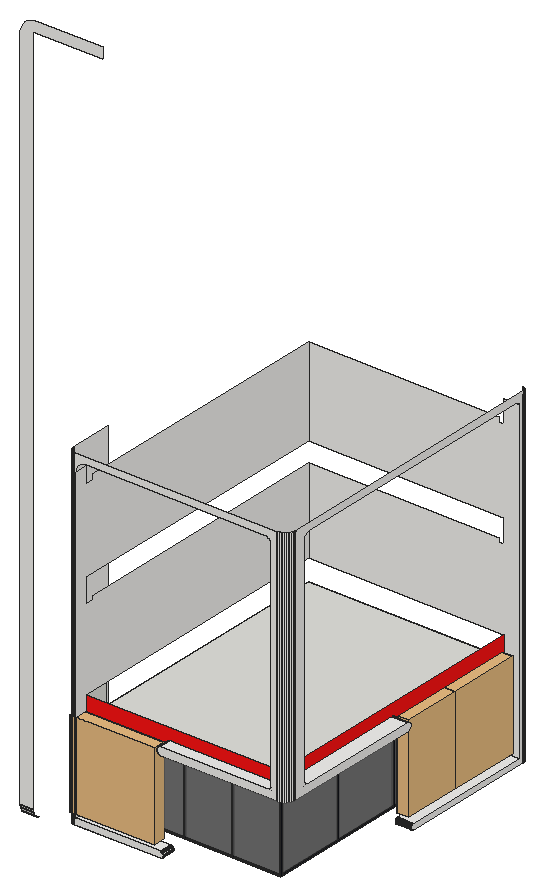
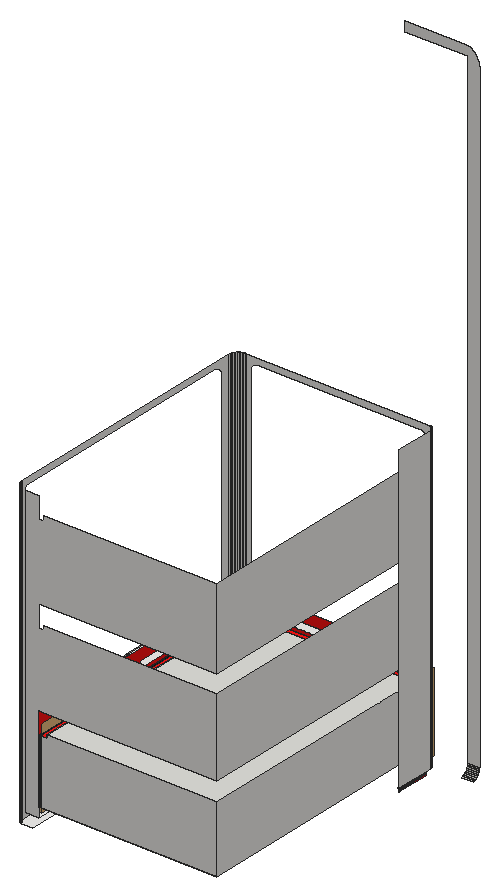
# SketchUp Ruby script. Lengths in inches.
U = 1.inch
M = Sketchup.active_model
def pt(a) = Geom::Point3d.new(a.map { |v| v * U })
def face(e, loops, mat)
  f = e.add_face(loops[0].map { |a| pt(a) })
  loops[1..].each { |l| e.add_face(l.map { |a| pt(a) }).erase! }
  f.material = f.back_material = mat if mat
  f
end
# faces: each face lists its corners as indices into pts; further lists are holes
def faces(e, pts, list, mat = nil) = list.each { |f| face(e, (f[0].is_a?(Array) ? f : [f]).map { |l| l.map { |i| pts[i] } }, mat) }
# xy, xz, yz: faces in a plane at the given z, y or x. An outline is a flat list of corners, or four numbers for a rectangle; further outlines are holes
def ring(l) = l.size == 4 ? [[l[0], l[1]], [l[2], l[1]], [l[2], l[3]], [l[0], l[3]]] : l.each_slice(2).to_a
def flat(e, list, mat, &to3) = list.each { |f| face(e, (f[0].is_a?(Array) ? f : [f]).map { |l| ring(l).map { |u, v| to3.(u, v) } }, mat) }
def xy(e, z, list, mat = nil) = flat(e, list, mat) { |x, y| [x, y, z] }
def xz(e, y, list, mat = nil) = flat(e, list, mat) { |x, z| [x, y, z] }
def yz(e, x, list, mat = nil) = flat(e, list, mat) { |y, z| [x, y, z] }
def lines(e, pts, list) = list.each { |a, b| e.add_line(pt(pts[a]), pt(pts[b])) }
# prism: a flat outline (further loops are holes) pulled along v
def prism(e, loops, v, mat = nil)
  f = face(e, loops, mat); d = Geom::Vector3d.new(v.map { |x| x * U })
  f.pushpull(f.normal.samedirection?(d) ? d.length : -d.length)
end
def box(e, o, s, mat = nil) = prism(e, [[o, [o[0] + s[0], o[1], o[2]], [o[0] + s[0], o[1] + s[1], o[2]], [o[0], o[1] + s[1], o[2]]]], [0, 0, s[2]], mat)
def at(x, y, z, deg = 0) = Geom::Transformation.translation(pt([x, y, z])) * Geom::Transformation.rotation(ORIGIN, Z_AXIS, deg.degrees)
def axes(o, x, y, z) = Geom::Transformation.new([*x, 0, *y, 0, *z, 0, *pt(o).to_a, 1])
def part(name) = M.definitions.add(name)
# library, detail: a bought-in or finely detailed component or shape, given as its bounding box
def library(name, o, s) = part(name).tap { |d| box(d.entities, o, s) }
def detail(e, o, s) = box(e.add_group.entities, o, s)
def put(e, d, t, mat = nil) = e.add_instance(d, t).tap { |i| i.material = mat if mat }
def group(e, t, mat = nil) = e.add_group.tap { |g| g.transformation = t; g.material = mat if mat }.entities
root = M.entities
M.materials.add("Generic").color = [242, 241, 238]
M.materials.add("Heather_Band").color = [255, 20, 20]
M.materials.add("Lisanne_Bandana").color = [222, 18, 34]
M.materials.add("{045efeae-c101-a24d-bd9b-6f5600100adb}").color = [102, 102, 102]
M.materials["{045efeae-c101-a24d-bd9b-6f5600100adb}"].alpha = 0.7
M.materials.add("{16756a1b-d383-d94f-ad82-104813d2624f}").color = [19, 21, 27]
c1 = library("Shrub+_Grass",[-121.83,-22.34,0],[123.96,19.94,123.95])
c2 = part("Furniture_0DcpanrIvuI8n_9Ae92L5A")
g1 = group(c2.entities,at(0,0,0))
box(g1,[-19.29,-0.2,0.39],[38.58,0.4,83.86],"{045efeae-c101-a24d-bd9b-6f5600100adb}")
g2 = group(c2.entities,at(0,0,0))
box(g2,[-19.68,-0.59,63.39],[39.36,1.18,0.39],"{16756a1b-d383-d94f-ad82-104813d2624f}")
box(g2,[-19.68,-0.59,42.52],[39.36,1.18,0.39],"{16756a1b-d383-d94f-ad82-104813d2624f}")
box(g2,[-19.68,-0.59,21.26],[39.36,1.18,0.39],"{16756a1b-d383-d94f-ad82-104813d2624f}")
xy(g2,0,[[-19.68,-0.59,19.68,0.59]],"{16756a1b-d383-d94f-ad82-104813d2624f}")
xy(g2,0.39,[[-19.68,-0.59,-19.29,0.59],[-19.68,-0.59,19.68,0.59],[19.29,-0.59,19.68,0.59]],"{16756a1b-d383-d94f-ad82-104813d2624f}")
xy(g2,84.25,[[-19.68,-0.59,19.68,0.59]],"{16756a1b-d383-d94f-ad82-104813d2624f}")
xy(g2,84.65,[[-19.68,-0.59,-19.29,0.59],[-19.68,-0.59,19.68,0.59],[19.29,-0.59,19.68,0.59]],"{16756a1b-d383-d94f-ad82-104813d2624f}")
xz(g2,-0.59,[[-19.68,0,19.68,0.39],[-19.68,0.39,-19.29,84.65],[19.29,0.39,19.68,84.65],[-19.68,84.25,19.68,84.65]],"{16756a1b-d383-d94f-ad82-104813d2624f}")
xz(g2,0.59,[[-19.68,0,19.68,0.39],[-19.68,0.39,-19.29,84.65],[19.29,0.39,19.68,84.65],[-19.68,84.25,19.68,84.65]],"{16756a1b-d383-d94f-ad82-104813d2624f}")
yz(g2,-19.68,[[-0.59,0,0.59,0.39],[-0.59,0.39,0.59,84.65],[-0.59,84.25,0.59,84.65]],"{16756a1b-d383-d94f-ad82-104813d2624f}")
yz(g2,-19.29,[[-0.59,0.39,0.59,84.65]],"{16756a1b-d383-d94f-ad82-104813d2624f}")
yz(g2,19.29,[[-0.59,0.39,0.59,84.65]],"{16756a1b-d383-d94f-ad82-104813d2624f}")
yz(g2,19.68,[[-0.59,0,0.59,0.39],[-0.59,0.39,0.59,84.65],[-0.59,84.25,0.59,84.65]],"{16756a1b-d383-d94f-ad82-104813d2624f}")
c3 = part("Glass+Window")
put(c3.entities,c2,at(0,0,-42.32))
xy(root,260.43,[[144.5,115.9,143.11,115.99,141.75,116.26,140.43,116.71,139.18,117.33,138.02,118.1,136.98,119.02,136.06,120.0625,135.28,121.22,134.67,122.47,134.22,123.79,133.95,125.15,133.86,126.54,133.86,200.9,136.89,200.9,136.89,137.375,291.875,137.375,291.875,115.9],[482.71,389.19,482.71,632.34,503.14,632.34,504.14,632.27,505.13,632.08,506.08,631.75,506.98,631.31,507.82,630.75,508.58,630.08,509.24,629.33,509.8,628.49,510.25,627.59,510.57,626.63,510.77,625.65,510.83,624.64,510.83,389.19]],"Generic")
xy(root,270.68,[[482.71,389.19,510.83,617.58]],"Generic")
xy(root,270.88,[[145.77,115.9,291.875,137.375]],"Generic")
xy(root,289.68,[[145.77,137.375,479.5,137.375,479.92,137.4,480.33,137.49,480.73,137.62,481.11,137.81,481.46,138.04,481.77,138.32,482.05,138.63,482.28,138.98,482.47,139.36,482.6,139.75,482.6875,140.17,482.71,140.59,482.71,617.58,145.77,617.58]])
xy(root,412.09,[[145.77,137.375,145.77,151.79,468.61,151.79,468.61,617.58,482.71,617.58,482.71,137.375]],"Heather_Band")
xy(root,416.32,[[145.77,151.79,468.61,617.58]])
xy(root,418.86,[[292.72,115.9,292.72,137.375,482.71,137.375,482.71,374.78,510.83,374.78,510.83,134.62,510.67,132.17,510.2,129.77,509.41,127.45,508.33,125.26,506.97,123.22,505.35,121.38,503.51,119.77,501.48,118.41,499.28,117.33,496.96,116.54,494.5625,116.0625,492.12,115.9]],"Generic")
xy(root,432.33,[[292.72,115.9,477.39,137.375],[482.71,160.35,510.83,374.78]],"Generic")
xz(root,96.24,[[65.42,274,87.56,274,87.56,1474.125,207.5,1474.125,207.5,1492.875,95.21,1492.875,91.33,1492.62,87.5,1491.86,83.8125,1490.61,80.32,1488.88,77.08,1486.72,74.15,1484.15,71.58,1481.22,69.41,1477.98,67.6875,1474.48,66.4375,1470.79,65.68,1466.97,65.42,1463.08]],"Generic")
xz(root,115.9,[[144.5,260.43,291.875,260.43,292.42,260.46,292.96,260.55,293.49,260.6875,294,260.89,294.49,261.13,294.95,261.43,295.37,261.78,295.76,262.16,296.1,262.59,296.4,263.05,296.65,263.53,296.84,264.04,296.99,264.57,297.07,265.11,297.1,265.66,297.07,266.2,296.99,266.74,296.84,267.27,296.65,267.78,296.4,268.27,296.1,268.73,295.76,269.15,295.37,269.54,294.95,269.88,294.49,270.18,294,270.43,293.49,270.625,292.96,270.77,292.42,270.85,291.875,270.88,145.77,270.88,145.77,805.02,145.93,807.42,146.39,809.78,147.17,812.05,148.23,814.21,149.5625,816.21,151.15,818.01,152.95,819.6,154.95,820.93,157.11,821.99,159.38,822.77,161.74,823.23,164.14,823.39,470.91,823.39,472.35,823.3,473.77,823.04,475.14,822.61,476.46,822.02,477.69,821.27,478.82,820.37,479.84,819.35,480.72,818.21,481.46,816.97,482.04,815.65,482.46,814.27,482.71,812.85,482.71,439.07,482.63,438.03,482.4,437,482.01,436.03,481.48,435.12,480.82,434.3,480.04,433.6,479.17,433.01,478.21,432.57,477.39,432.33,292.72,432.33,292.02,432.29,291.32,432.18,290.64,432,289.98,431.75,289.35,431.43,288.76,431.04,288.21,430.6,287.71,430.1,287.27,429.55,286.89,428.96,286.57,428.33,286.3125,427.68,286.13,426.99,286.02,426.3,285.98,425.59,286.02,424.89,286.13,424.19,286.3125,423.51,286.57,422.85,286.89,422.23,287.27,421.63,287.71,421.09,288.21,420.59,288.76,420.14,289.35,419.76,289.98,419.4375,290.64,419.1875,291.32,419,292.02,418.89,292.72,418.86,492.12,418.86,492.12,835.52,144.5,835.52]],"Generic")
xz(root,137.375,[[145.77,412.09,482.71,412.09,482.71,418.86,292.72,418.86,292.02,418.89,291.32,419,290.64,419.1875,289.98,419.4375,289.35,419.76,288.76,420.14,288.21,420.59,287.71,421.09,287.27,421.63,286.89,422.23,286.57,422.85,286.3125,423.51,286.13,424.19,286.02,424.89,285.98,425.59,286.02,426.3,286.13,426.99,286.3125,427.68,286.57,428.33,286.89,428.96,287.27,429.55,287.71,430.1,288.21,430.6,288.76,431.04,289.35,431.43,289.98,431.75,290.64,432,291.32,432.18,292.02,432.29,292.72,432.33,477.39,432.33,478.21,432.57,479.17,433.01,480.04,433.6,480.82,434.3,481.48,435.12,482.01,436.03,482.4,437,482.63,438.03,482.71,439.07,482.71,452.24,145.77,452.24]],"Heather_Band")
xz(root,151.79,[[145.77,412.09,468.61,416.32]])
xz(root,617.58,[[482.71,270.68,510.83,270.68,510.83,817.55,482.71,817.55,482.71,777.77,474.55,777.77,474.55,786.62,145.77,786.62,145.77,633.64,482.71,633.64,482.71,592.96,474.55,592.96,474.55,599,145.77,599,145.77,452.24,482.71,452.24,482.71,412.09,468.61,412.09,468.61,416.32,145.77,416.32,145.77,289.68,482.71,289.68]],"Generic")
yz(root,133.86,[[126.54,260.43,200.9,835.52]],"Generic")
yz(root,133.86,[[137.375,255.93,200.9,255.95],[137.375,255.95,200.9,257.23]],"Lisanne_Bandana")
yz(root,145.77,[[137.375,412.09,151.79,412.09,151.79,416.32,181.19,416.32,180.67,452.24,137.375,452.24]])
yz(root,145.77,[[115.9,270.88,137.375,270.88,137.375,289.68,617.58,289.68,617.58,416.32,151.79,416.32,151.79,412.09,137.375,412.09,137.375,452.24,617.58,452.24,617.58,599,151.79,599,151.79,592.96,137.375,592.96,137.375,633.64,617.58,633.64,617.58,786.62,151.79,786.62,151.79,777.77,137.375,777.77,137.375,805.02,115.9,805.02]],"Generic")
yz(root,468.61,[[151.79,412.09,617.58,416.32]])
yz(root,482.71,[[137.375,412.09,617.58,412.09,617.58,452.24,150.43,452.24,150.43,444.64,150.51,443.22,150.75,441.82,151.15,440.45,151.69,439.14,152.39,437.89,153.22,436.74,154.17,435.68,155.24,434.74,156.41,433.92,157.66,433.24,158.98,432.71,160.35,432.33,374.78,432.33,375.48,432.29,376.18,432.18,376.86,432,377.52,431.75,378.15,431.43,378.74,431.04,379.29,430.6,379.78,430.1,380.23,429.55,380.61,428.96,380.93,428.33,381.18,427.68,381.37,426.99,381.48,426.3,381.51,425.59,381.48,424.89,381.37,424.19,381.18,423.51,380.93,422.85,380.61,422.23,380.23,421.63,379.78,421.09,379.29,420.59,378.74,420.14,378.15,419.76,377.52,419.4375,376.86,419.1875,376.18,419,375.48,418.89,374.78,418.86,137.375,418.86]],"Heather_Band")
yz(root,510.83,[[389.19,260.43,624.64,260.43,624.64,835.52,134.62,835.52,134.62,418.86,374.78,418.86,375.48,418.89,376.18,419,376.86,419.1875,377.52,419.4375,378.15,419.76,378.74,420.14,379.29,420.59,379.78,421.09,380.23,421.63,380.61,422.23,380.93,422.85,381.18,423.51,381.37,424.19,381.48,424.89,381.51,425.59,381.48,426.3,381.37,426.99,381.18,427.68,380.93,428.33,380.61,428.96,380.23,429.55,379.78,430.1,379.29,430.6,378.74,431.04,378.15,431.43,377.52,431.75,376.86,432,376.18,432.18,375.48,432.29,374.78,432.33,160.35,432.33,158.98,432.71,157.66,433.24,156.41,433.92,155.24,434.74,154.17,435.68,153.22,436.74,152.39,437.89,151.69,439.14,151.15,440.45,150.75,441.82,150.51,443.22,150.43,444.64,150.43,812.2,150.69,813.56,151.33,815.38,152.22,817.09,153.35,818.65,154.7,820.04,156.23,821.21,157.92,822.15,159.72,822.83,161.6,823.25,163.53,823.39,611.74,823.39,612.51,823.34,613.26,823.19,613.98,822.95,614.66,822.61,615.3,822.18,615.875,821.68,616.38,821.11,616.8,820.47,617.14,819.79,617.39,819.0625,617.53,818.3125,617.58,817.55,617.58,270.68,389.19,270.68,388.71,270.58,388.25,270.43,387.79,270.25,387.36,270.02,386.95,269.75,386.57,269.45,386.22,269.11,385.9,268.73,385.625,268.33,385.38,267.91,385.18,267.46,385.02,267,384.91,266.53,384.84,266.04,384.82,265.56,384.84,265.07,384.91,264.58,385.02,264.11,385.18,263.65,385.38,263.2,385.625,262.78,385.9,262.375,386.22,262.01,386.57,261.67,386.95,261.36,387.36,261.09,387.79,260.86,388.25,260.68,388.71,260.53]],"Generic")
p = [[134.74,137.375,254.14],[134.18,137.375,254.98],[134.18,200.9,254.98],[134.74,200.9,254.14],[87.56,109.26,254.51],[87.56,106.79,255.73],
  [65.42,106.79,255.73],[65.42,109.26,254.51],[133.86,137.375,255.93],[133.86,200.9,255.93],[87.56,104.49,257.26],[65.42,104.49,257.26],
  [133.86,137.375,257.23],[133.99,137.375,257.91],[133.99,200.9,257.91],[133.86,200.9,257.23],[87.56,102.42,259.08],[65.42,102.42,259.08],
  [134.44,137.375,258.81],[134.44,200.9,258.81],[135.1,137.375,259.56],[135.1,200.9,259.56],[87.56,100.6,261.16],[65.42,100.6,261.16],
  [135.9375,137.375,260.11],[135.9375,200.9,260.11],[136.89,137.375,260.43],[136.89,200.9,260.43],[144.5,115.9,835.52],[143.11,115.99,835.52],
  [143.11,115.99,260.43],[144.5,115.9,260.43],[292.42,115.9,260.46],[291.875,115.9,260.43],[291.875,137.375,260.43],[292.42,137.375,260.46],
  [141.75,116.26,835.52],[141.75,116.26,260.43],[140.43,116.71,835.52],[140.43,116.71,260.43],[139.18,117.33,835.52],[139.18,117.33,260.43],
  [138.02,118.1,835.52],[138.02,118.1,260.43],[136.98,119.02,835.52],[136.98,119.02,260.43],[136.06,120.0625,835.52],[136.06,120.0625,260.43],
  [135.28,121.22,835.52],[135.28,121.22,260.43],[134.67,122.47,835.52],[134.67,122.47,260.43],[134.22,123.79,835.52],[134.22,123.79,260.43],
  [133.95,125.15,835.52],[133.95,125.15,260.43],[133.86,126.54,835.52],[133.86,126.54,260.43],[510.83,389.19,260.43],[510.83,388.71,260.53],
  [482.71,388.71,260.53],[482.71,389.19,260.43],[510.77,625.65,835.52],[510.83,624.64,835.52],[510.83,624.64,260.43],[510.77,625.65,260.43],
  [510.57,626.63,835.52],[510.57,626.63,260.43],[510.25,627.59,835.52],[510.25,627.59,260.43],[509.8,628.49,835.52],[509.8,628.49,260.43],
  [509.24,629.33,835.52],[509.24,629.33,260.43],[508.58,630.08,835.52],[508.58,630.08,260.43],[507.82,630.75,835.52],[507.82,630.75,260.43],
  [506.98,631.31,835.52],[506.98,631.31,260.43],[506.08,631.75,835.52],[506.08,631.75,260.43],[505.13,632.08,835.52],[505.13,632.08,260.43],
  [504.14,632.27,835.52],[504.14,632.27,260.43],[503.14,632.34,835.52],[503.14,632.34,260.43],[292.96,115.9,260.55],[292.96,137.375,260.55],
  [293.49,115.9,260.6875],[293.49,137.375,260.6875],[510.83,388.25,260.68],[482.71,388.25,260.68],[294,115.9,260.89],[294,137.375,260.89],
  [510.83,387.79,260.86],[482.71,387.79,260.86],[294.49,115.9,261.13],[294.49,137.375,261.13],[510.83,387.36,261.09],[482.71,387.36,261.09],
  [294.95,115.9,261.43],[294.95,137.375,261.43],[510.83,386.95,261.36],[482.71,386.95,261.36],[87.56,99.07,263.45],[65.42,99.07,263.45],
  [295.37,115.9,261.78],[295.37,137.375,261.78],[510.83,386.57,261.67],[482.71,386.57,261.67],[510.83,386.22,262.01],[482.71,386.22,262.01],
  [295.76,115.9,262.16],[295.76,137.375,262.16],[510.83,385.9,262.375],[482.71,385.9,262.375],[296.1,115.9,262.59],[296.1,137.375,262.59],
  [510.83,385.625,262.78],[482.71,385.625,262.78],[296.4,115.9,263.05],[296.4,137.375,263.05],[510.83,385.38,263.2],[482.71,385.38,263.2],
  [296.65,115.9,263.53],[296.65,137.375,263.53],[510.83,385.18,263.65],[482.71,385.18,263.65],[87.56,97.85,265.93],[65.42,97.85,265.93],
  [296.84,115.9,264.04],[296.84,137.375,264.04],[510.83,385.02,264.11],[482.71,385.02,264.11],[296.99,115.9,264.57],[296.99,137.375,264.57],
  [510.83,384.91,264.58],[482.71,384.91,264.58],[297.07,115.9,265.11],[297.07,137.375,265.11],[510.83,384.84,265.07],[482.71,384.84,265.07],
  [297.1,115.9,265.66],[297.1,137.375,265.66],[510.83,384.82,265.56],[482.71,384.82,265.56],[510.83,384.84,266.04],[482.71,384.84,266.04],
  [297.07,115.9,266.2],[297.07,137.375,266.2],[87.56,96.96,268.54],[65.42,96.96,268.54],[510.83,384.91,266.53],[482.71,384.91,266.53],
  [296.99,115.9,266.74],[296.99,137.375,266.74],[510.83,385.02,267],[482.71,385.02,267],[296.84,115.9,267.27],[296.84,137.375,267.27],
  [510.83,385.18,267.46],[482.71,385.18,267.46],[296.65,115.9,267.78],[296.65,137.375,267.78],[510.83,385.38,267.91],[482.71,385.38,267.91],
  [296.4,115.9,268.27],[296.4,137.375,268.27],[510.83,385.625,268.33],[482.71,385.625,268.33],[296.1,115.9,268.73],[296.1,137.375,268.73],
  [510.83,385.9,268.73],[482.71,385.9,268.73],[87.56,96.42,271.25],[65.42,96.42,271.25],[295.76,115.9,269.15],[295.76,137.375,269.15],
  [510.83,386.22,269.11],[482.71,386.22,269.11],[510.83,386.57,269.45],[482.71,386.57,269.45],[295.37,115.9,269.54],[295.37,137.375,269.54],
  [510.83,386.95,269.75],[482.71,386.95,269.75],[294.95,115.9,269.88],[294.95,137.375,269.88],[510.83,387.36,270.02],[482.71,387.36,270.02],
  [294.49,115.9,270.18],[294.49,137.375,270.18],[510.83,387.79,270.25],[482.71,387.79,270.25],[294,115.9,270.43],[294,137.375,270.43],
  [510.83,388.25,270.43],[482.71,388.25,270.43],[293.49,115.9,270.625],[293.49,137.375,270.625],[510.83,388.71,270.58],[482.71,388.71,270.58],
  [292.96,115.9,270.77],[292.96,137.375,270.77],[510.83,389.19,270.68],[482.71,389.19,270.68],[292.42,115.9,270.85],[292.42,137.375,270.85],
  [291.875,115.9,270.88],[291.875,137.375,270.88],[87.56,96.24,274],[65.42,96.24,274],[292.02,115.9,418.89],[291.32,115.9,419],
  [291.32,137.375,419],[292.02,137.375,418.89],[292.72,115.9,418.86],[292.72,137.375,418.86],[494.5625,116.0625,835.52],[492.12,115.9,835.52],
  [492.12,115.9,418.86],[494.5625,116.0625,418.86],[496.96,116.54,835.52],[496.96,116.54,418.86],[499.28,117.33,835.52],[499.28,117.33,418.86],
  [501.48,118.41,835.52],[501.48,118.41,418.86],[503.51,119.77,835.52],[503.51,119.77,418.86],[505.35,121.38,835.52],[505.35,121.38,418.86],
  [506.97,123.22,835.52],[506.97,123.22,418.86],[508.33,125.26,835.52],[508.33,125.26,418.86],[509.41,127.45,835.52],[509.41,127.45,418.86],
  [510.2,129.77,835.52],[510.2,129.77,418.86],[510.67,132.17,835.52],[510.67,132.17,418.86],[510.83,134.62,835.52],[510.83,134.62,418.86],
  [510.83,375.48,418.89],[510.83,374.78,418.86],[482.71,374.78,418.86],[482.71,375.48,418.89],[510.83,376.18,419],[482.71,376.18,419],
  [290.64,115.9,419.1875],[290.64,137.375,419.1875],[510.83,376.86,419.1875],[482.71,376.86,419.1875],[289.98,115.9,419.4375],[289.98,137.375,419.4375],
  [510.83,377.52,419.4375],[482.71,377.52,419.4375],[289.35,115.9,419.76],[289.35,137.375,419.76],[510.83,378.15,419.76],[482.71,378.15,419.76],
  [288.76,115.9,420.14],[288.76,137.375,420.14],[510.83,378.74,420.14],[482.71,378.74,420.14],[288.21,115.9,420.59],[288.21,137.375,420.59],
  [510.83,379.29,420.59],[482.71,379.29,420.59],[287.71,115.9,421.09],[287.71,137.375,421.09],[510.83,379.78,421.09],[482.71,379.78,421.09],
  [287.27,115.9,421.63],[287.27,137.375,421.63],[510.83,380.23,421.63],[482.71,380.23,421.63],[286.89,115.9,422.23],[286.89,137.375,422.23],
  [510.83,380.61,422.23],[482.71,380.61,422.23],[286.57,115.9,422.85],[286.57,137.375,422.85],[510.83,380.93,422.85],[482.71,380.93,422.85],
  [286.3125,115.9,423.51],[286.3125,137.375,423.51],[510.83,381.18,423.51],[482.71,381.18,423.51],[286.13,115.9,424.19],[286.13,137.375,424.19],
  [510.83,381.37,424.19],[482.71,381.37,424.19],[286.02,115.9,424.89],[286.02,137.375,424.89],[510.83,381.48,424.89],[482.71,381.48,424.89],
  [285.98,115.9,425.59],[285.98,137.375,425.59],[510.83,381.51,425.59],[482.71,381.51,425.59],[286.02,115.9,426.3],[286.02,137.375,426.3],
  [510.83,381.48,426.3],[482.71,381.48,426.3],[286.13,115.9,426.99],[286.13,137.375,426.99],[510.83,381.37,426.99],[482.71,381.37,426.99],
  [286.3125,115.9,427.68],[286.3125,137.375,427.68],[510.83,381.18,427.68],[482.71,381.18,427.68],[286.57,115.9,428.33],[286.57,137.375,428.33],
  [510.83,380.93,428.33],[482.71,380.93,428.33],[286.89,115.9,428.96],[286.89,137.375,428.96],[510.83,380.61,428.96],[482.71,380.61,428.96],
  [287.27,115.9,429.55],[287.27,137.375,429.55],[510.83,380.23,429.55],[482.71,380.23,429.55],[287.71,115.9,430.1],[287.71,137.375,430.1],
  [510.83,379.78,430.1],[482.71,379.78,430.1],[288.21,115.9,430.6],[288.21,137.375,430.6],[510.83,379.29,430.6],[482.71,379.29,430.6],
  [288.76,115.9,431.04],[288.76,137.375,431.04],[510.83,378.74,431.04],[482.71,378.74,431.04],[289.35,115.9,431.43],[289.35,137.375,431.43],
  [510.83,378.15,431.43],[482.71,378.15,431.43],[289.98,115.9,431.75],[289.98,137.375,431.75],[510.83,377.52,431.75],[482.71,377.52,431.75],
  [290.64,115.9,432],[290.64,137.375,432],[510.83,376.86,432],[482.71,376.86,432],[291.32,115.9,432.18],[291.32,137.375,432.18],
  [510.83,376.18,432.18],[482.71,376.18,432.18],[292.02,115.9,432.29],[292.02,137.375,432.29],[510.83,375.48,432.29],[482.71,375.48,432.29],
  [292.72,115.9,432.33],[292.72,137.375,432.33],[477.39,115.9,432.33],[478.21,115.9,432.57],[478.21,137.375,432.57],[477.39,137.375,432.33],
  [510.83,158.98,432.71],[510.83,160.35,432.33],[482.71,160.35,432.33],[482.71,158.98,432.71],[510.83,374.78,432.33],[482.71,374.78,432.33],
  [479.17,115.9,433.01],[479.17,137.375,433.01],[510.83,157.66,433.24],[482.71,157.66,433.24],[480.04,115.9,433.6],[480.04,137.375,433.6],
  [510.83,156.41,433.92],[482.71,156.41,433.92],[480.82,115.9,434.3],[480.82,137.375,434.3],[510.83,155.24,434.74],[482.71,155.24,434.74],
  [481.48,115.9,435.12],[481.48,137.375,435.12],[510.83,154.17,435.68],[482.71,154.17,435.68],[482.01,115.9,436.03],[482.01,137.375,436.03],
  [482.71,150.43,432.33],[482.71,115.9,432.33],[482.71,137.375,432.33],[482.71,137.375,439.07],[510.83,150.43,432.33],[482.71,150.43,444.64]]
faces(root,p,[[0,1,2,3],[1,8,9,2],[12,13,14,15],[13,18,19,14],[18,20,21,19],[20,24,25,21],[24,26,27,25]],"Lisanne_Bandana")
faces(root,p,[[4,5,6,7],[5,10,11,6],[10,16,17,11],[16,22,23,17],[28,29,30,31],[32,33,34,35],[29,36,37,30],[36,38,39,37],
  [38,40,41,39],[40,42,43,41],[42,44,45,43],[44,46,47,45],[46,48,49,47],[48,50,51,49],[50,52,53,51],[52,54,55,53],
  [54,56,57,55],[58,59,60,61],[62,63,64,65],[66,62,65,67],[68,66,67,69],[70,68,69,71],[72,70,71,73],[74,72,73,75],
  [76,74,75,77],[78,76,77,79],[80,78,79,81],[82,80,81,83],[84,82,83,85],[86,84,85,87],[88,32,35,89],[90,88,89,91],
  [59,92,93,60],[94,90,91,95],[92,96,97,93],[98,94,95,99],[96,100,101,97],[102,98,99,103],[100,104,105,101],[22,106,107,23],
  [108,102,103,109],[104,110,111,105],[110,112,113,111],[114,108,109,115],[112,116,117,113],[118,114,115,119],[116,120,121,117],[122,118,119,123],
  [120,124,125,121],[126,122,123,127],[124,128,129,125],[106,130,131,107],[132,126,127,133],[128,134,135,129],[136,132,133,137],[134,138,139,135],
  [140,136,137,141],[138,142,143,139],[144,140,141,145],[142,146,147,143],[146,148,149,147],[150,144,145,151],[130,152,153,131],[148,154,155,149],
  [156,150,151,157],[154,158,159,155],[160,156,157,161],[158,162,163,159],[164,160,161,165],[162,166,167,163],[168,164,165,169],[166,170,171,167],
  [172,168,169,173],[170,174,175,171],[152,176,177,153],[178,172,173,179],[174,180,181,175],[180,182,183,181],[184,178,179,185],[182,186,187,183],
  [188,184,185,189],[186,190,191,187],[192,188,189,193],[190,194,195,191],[196,192,193,197],[194,198,199,195],[200,196,197,201],[198,202,203,199],
  [204,200,201,205],[202,206,207,203],[208,204,205,209],[210,208,209,211],[176,212,213,177],[214,215,216,217],[218,214,217,219],[220,221,222,223],
  [224,220,223,225],[226,224,225,227],[228,226,227,229],[230,228,229,231],[232,230,231,233],[234,232,233,235],[236,234,235,237],[238,236,237,239],
  [240,238,239,241],[242,240,241,243],[244,242,243,245],[246,247,248,249],[250,246,249,251],[215,252,253,216],[254,250,251,255],[252,256,257,253],
  [258,254,255,259],[256,260,261,257],[262,258,259,263],[260,264,265,261],[266,262,263,267],[264,268,269,265],[270,266,267,271],[268,272,273,269],
  [274,270,271,275],[272,276,277,273],[278,274,275,279],[276,280,281,277],[282,278,279,283],[280,284,285,281],[286,282,283,287],[284,288,289,285],
  [290,286,287,291],[288,292,293,289],[294,290,291,295],[292,296,297,293],[298,294,295,299],[296,300,301,297],[302,298,299,303],[300,304,305,301],
  [306,302,303,307],[304,308,309,305],[310,306,307,311],[308,312,313,309],[314,310,311,315],[312,316,317,313],[318,314,315,319],[316,320,321,317],
  [322,318,319,323],[320,324,325,321],[326,322,323,327],[324,328,329,325],[330,326,327,331],[328,332,333,329],[334,330,331,335],[332,336,337,333],
  [338,334,335,339],[336,340,341,337],[342,338,339,343],[340,344,345,341],[346,342,343,347],[344,348,349,345],[350,346,347,351],[348,352,353,349],
  [354,350,351,355],[352,356,357,353],[358,354,355,359],[356,360,361,357],[362,363,364,365],[366,367,368,369],[370,358,359,371],[363,372,373,364],
  [374,366,369,375],[372,376,377,373],[378,374,375,379],[376,380,381,377],[382,378,379,383],[380,384,385,381],[386,382,383,387],[384,388,389,385]],"Generic")
lines(root,p,[[390,368],[391,392],[393,392],[365,392],[394,390],[395,390]])
put(root,c1,axes([279.6875,138.24,277.13],[1.1844,0,0],[0,1,0],[0,0,1.21]))
put(root,c1,axes([479.68,610.4,277.96],[0,1,0],[-1,0,0],[0,0,1.21]))
put(root,c1,axes([479.68,486.81,277.96],[0,0.81,0],[-1,0,0],[0,0,1.21]))
put(root,c3,axes([314.24,138.68,350.59],[0,0,-3.09427],[0,2.2,0],[3.98066,0,0]),"Heather_Band")
put(root,c3,axes([481.41,378.78,350.89],[0,0,-3.10921],[-2.2,0,0],[0,5.64246,0]),"Heather_Band")
